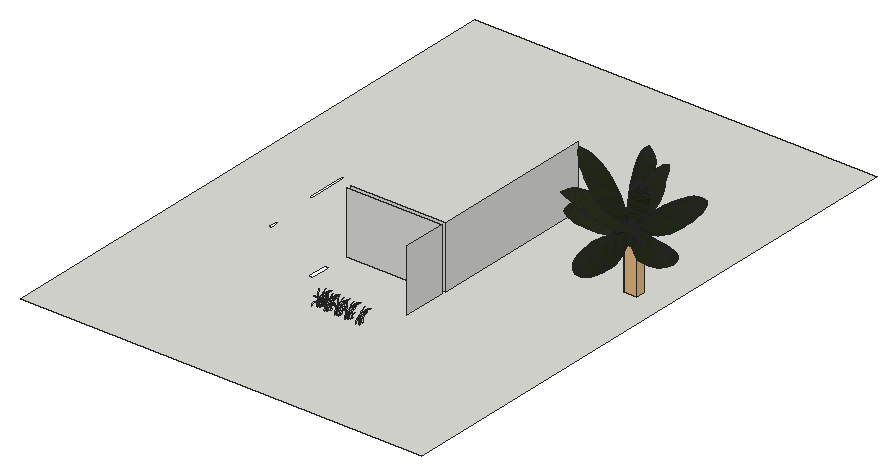
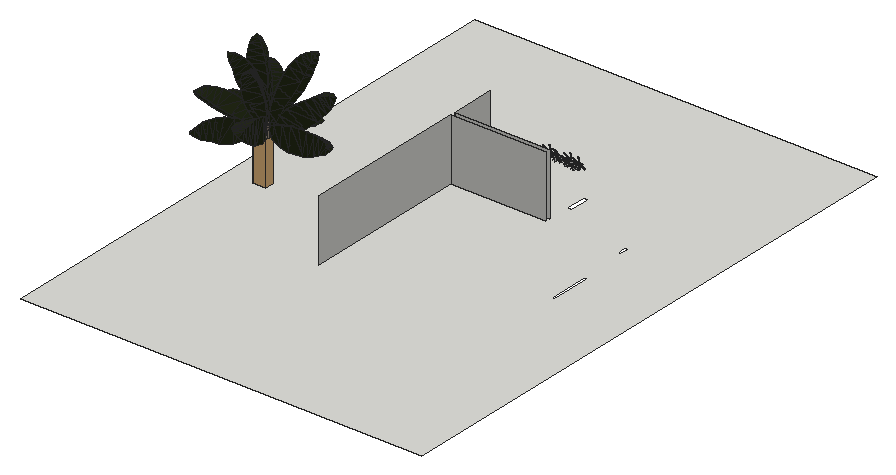
# SketchUp Ruby script. Lengths in inches.
U = 1.inch
M = Sketchup.active_model
def pt(a) = Geom::Point3d.new(a.map { |v| v * U })
def face(e, loops, mat)
  f = e.add_face(loops[0].map { |a| pt(a) })
  loops[1..].each { |l| e.add_face(l.map { |a| pt(a) }).erase! }
  f.material = f.back_material = mat if mat
  f
end
# faces: each face lists its corners as indices into pts; further lists are holes
def faces(e, pts, list, mat = nil) = list.each { |f| face(e, (f[0].is_a?(Array) ? f : [f]).map { |l| l.map { |i| pts[i] } }, mat) }
# xy, xz, yz: faces in a plane at the given z, y or x. An outline is a flat list of corners, or four numbers for a rectangle; further outlines are holes
def ring(l) = l.size == 4 ? [[l[0], l[1]], [l[2], l[1]], [l[2], l[3]], [l[0], l[3]]] : l.each_slice(2).to_a
def flat(e, list, mat, &to3) = list.each { |f| face(e, (f[0].is_a?(Array) ? f : [f]).map { |l| ring(l).map { |u, v| to3.(u, v) } }, mat) }
def xy(e, z, list, mat = nil) = flat(e, list, mat) { |x, y| [x, y, z] }
def xz(e, y, list, mat = nil) = flat(e, list, mat) { |x, z| [x, y, z] }
def yz(e, x, list, mat = nil) = flat(e, list, mat) { |y, z| [x, y, z] }
def lines(e, pts, list) = list.each { |a, b| e.add_line(pt(pts[a]), pt(pts[b])) }
# prism: a flat outline (further loops are holes) pulled along v
def prism(e, loops, v, mat = nil)
  f = face(e, loops, mat); d = Geom::Vector3d.new(v.map { |x| x * U })
  f.pushpull(f.normal.samedirection?(d) ? d.length : -d.length)
end
def box(e, o, s, mat = nil) = prism(e, [[o, [o[0] + s[0], o[1], o[2]], [o[0] + s[0], o[1] + s[1], o[2]], [o[0], o[1] + s[1], o[2]]]], [0, 0, s[2]], mat)
def at(x, y, z, deg = 0) = Geom::Transformation.translation(pt([x, y, z])) * Geom::Transformation.rotation(ORIGIN, Z_AXIS, deg.degrees)
def axes(o, x, y, z) = Geom::Transformation.new([*x, 0, *y, 0, *z, 0, *pt(o).to_a, 1])
def part(name) = M.definitions.add(name)
# library, detail: a bought-in or finely detailed component or shape, given as its bounding box
def library(name, o, s) = part(name).tap { |d| box(d.entities, o, s) }
def detail(e, o, s) = box(e.add_group.entities, o, s)
def put(e, d, t, mat = nil) = e.add_instance(d, t).tap { |i| i.material = mat if mat }
def group(e, t, mat = nil) = e.add_group.tap { |g| g.transformation = t; g.material = mat if mat }.entities
root = M.entities
M.materials.add("cocoanut_mat").color = [137, 122, 109]
M.materials.add("cocoanut_scrub").color = [165, 152, 134]
M.materials.add("coconut_test3_clean").color = [38, 45, 24]
c1 = part("coconut_half")
p = [[54.48,2.6,2.17],[90.24,0,0],[105.09,35.75,42.48],[115.87,5,0],[128.48,35.75,36.0625],[152.37,21,0],
  [152.37,35.75,27.13],[169.19,35.75,17.77],[57.93,35.75,46.59],[42.36,5.25,5.16],[79.93,35.75,46.59],[41.85,35.75,44.23],
  [28.04,8.5,7.49],[27.85,35.75,39.58],[16.59,14.5,9.63],[9.27,35.75,26.98],[6.26,23.5,11.78],[16.71,35.75,32.89],
  [0,35.75,14.25]]
faces(c1.entities,p,[[0,1,2],[1,3,4],[1,4,2],[3,5,6],[3,6,4],[5,7,6],[0,8,9],[0,10,8],
  [0,2,10],[9,11,12],[9,8,11],[12,13,14],[12,11,13],[14,15,16],[14,17,15],[14,13,17],
  [18,16,15]],"coconut_test3_clean")
c2 = part("Group\#44")
put(c2.entities,c1,at(0,0,0))
put(c2.entities,c1,axes([0,71.5,0],[1,0,0],[0,-1,0],[0,0,1]))
c3 = part("coconut3_top")
put(c3.entities,c2,axes([-176.42,-40.5625,245.57],[1,0,0],[0,0.96593,-0.25882],[0,0.25882,0.96593]))
g1 = group(c3.entities,at(-4.7,-151.6,178.32))
put(g1,c1,axes([0,0,0],[0.14944,0.9543,0.25882],[-0.87562,0.00613,0.48296],[0.4593,-0.2988,0.83652]))
put(g1,c1,axes([-62.61,0.4375,34.53],[0.14944,0.9543,0.25882],[0.87562,-0.00613,-0.48296],[0.4593,-0.2988,0.83652]))
put(c3.entities,c2,axes([171.02,-15.64,245.06],[-0.94665,0.32227,0],[-0.31128,-0.91439,-0.25882],[-0.08341,-0.24501,0.96593]))
put(c3.entities,c2,axes([41.29,183.8,264.73],[-0.39574,-0.90582,-0.15126],[0.91636,-0.40035,0],[-0.06056,-0.13861,0.98849]))
put(c3.entities,c2,axes([-77.19,156.92,280.49],[0.30009,-0.91813,-0.25882],[0.86338,0.14605,0.48296],[-0.40562,-0.36839,0.83652]))
put(c3.entities,c2,axes([-112.56,-104.35,340.4],[0.76036,0.41456,-0.5],[-0.63406,0.64068,-0.43301],[0.14083,0.64627,0.75]))
put(c3.entities,c2,axes([119.49,-113.07,311.83],[-0.54618,0.67208,-0.5],[-0.83762,-0.43208,0.3342],[0.00857,0.60135,0.79894]))
put(c3.entities,c2,axes([103.27,116.54,337.13],[-0.75167,-0.49748,-0.43301],[0.65951,-0.56129,-0.5],[0.0057,-0.66141,0.75]))
put(c3.entities,c2,axes([-111.91,-75.47,434.48],[0.55528,0.30275,-1.09544],[-0.10884,0.68367,0.13377],[0.95166,0.05419,0.49738]))
put(c3.entities,c2,axes([96.22,-37.8,421.8],[-0.43628,0.34579,-0.96422],[-0.35338,-0.74638,-0.10777],[-0.75439,0.29273,0.44631]))
put(c3.entities,c2,axes([-41.59,80.66,420.02],[0.06101,-0.43197,-0.99256],[0.722,0.18761,-0.03727],[0.23024,-0.81295,0.36796]))
put(c3.entities,c2,axes([62.57,69.42,421.8],[-0.49424,-0.25619,-0.96422],[0.53593,-0.62829,-0.10777],[-0.57624,-0.5681,0.44631]))
c4 = part("cocoanut_mat")
yz(c4.entities,2,[[0.45,5,4.17,5,4.55,7.22,0,7.22]],"cocoanut_mat")
p = [[1.5,0.95,2.55],[0,1.26,0],[1.5,4.17,2.55],[0,3.01,0.06],[2,0.45,5],[2,4.17,5],
  [1.5,4.82,10.82],[1.5,0,9.97],[2,4.55,7.22],[2,0,7.22],[1,0.99,11.1],[1,3.98,11.36]]
faces(c4.entities,p,[[0,1,2],[3,2,1],[4,0,2,5],[6,7,8],[9,8,7],[7,6,10],[11,10,6]],"cocoanut_mat")
c5 = part("Coconut Palm")
xy(c5.entities,112.14,[[122.28,106.09,125.08,107.25,126.24,110.05,125.08,112.85,122.28,114.01,119.48,112.85,118.32,110.05,119.48,107.25]])
detail(c5.entities,[118.32,101.24,0],[25.61,17.45,83.17])
put(c5.entities,c3,axes([125.26,110.5,-76.06],[0.71,0,0],[0,0.71,0],[0,0,0.71]))
g2 = group(c5.entities,at(117.6,103.69,82.125))
p = [[4.68,2.4,1.05],[4.68,2.4,30.02],[1.88,3.56,30.02],[1.88,3.56,1.05],[7.48,3.56,1.05],[7.48,3.56,30.02],
  [0.72,6.36,30.02],[0.72,6.36,1.05],[8.64,6.36,1.05],[8.64,6.36,30.02],[1.88,9.16,30.02],[1.88,9.16,1.05],
  [7.48,9.16,1.05],[7.48,9.16,30.02],[4.68,10.32,30.02],[4.68,10.32,1.05]]
faces(g2,p,[[0,1,2,3],[4,5,1,0],[2,6,7,3],[4,8,9,5],[6,10,11,7],[8,12,13,9],[11,10,14,15],[15,14,13,12]],"cocoanut_scrub")
put(g2,c4,axes([8.73,9,14.81],[0.95137,0.17914,0.2506],[-0.24236,0.93742,0.25],[-0.19013,-0.29858,0.93525]))
put(g2,c4,axes([1.89,13.92,14.26],[-0.95388,0.23795,0.18301],[-0.27087,-0.94506,-0.18301],[0.17341,-0.30035,1.29434]))
put(g2,c4,axes([3.98,0.08,4.09],[0.521,-0.82169,0.23104],[0.85353,0.50368,-0.13339],[-0.00676,0.2667,0.96376]))
put(g2,c4,axes([2.8,2.4,6.76],[-0.16755,-0.98247,0.08171],[0.984,-0.16156,0.07513],[-0.09879,0.15157,1.61993]))
put(g2,c4,axes([8.29,10.47,4.97],[0.02489,0.99575,0.08868],[-0.99708,0.03112,-0.06968],[-0.11254,-0.13523,1.55005]))
put(g2,c4,axes([10.54,2.88,6.76],[0.95137,0.17914,0.2506],[-0.115,0.96125,-0.25056],[-0.28577,0.20956,0.9351]))
xy(root,0,[[[75.43,0,853.18,1102.0625],[219.74,518.03,227.09,597.83],[372.21,325.52,381.21,367.52],[229.21,408.6,235.21,426.23]]])
xz(root,409.52,[[381.21,0,565.21,120]])
xz(root,418.52,[[381.21,0,565.21,120]])
yz(root,565.21,[[325.52,0,409.52,120],[418.52,0,739.58,120]])
g3 = group(root,at(460.01,260.65,0))
p = [[-0.98,0.17,0],[-0.43,0.08,0],[0,0,1.75],[-0.18,0.03,3.51],[-0.96,0.17,5.24],[-2.32,0.41,6.89],
  [-4.24,0.76,8.42],[-6.67,1.1875,9.8],[-9.54,1.7,10.98],[-12.78,2.28,11.95],[-16.32,2.91,12.67],[-20.06,3.57,13.13],
  [-23.91,4.26,13.32],[-27.78,4.95,13.23],[-23.98,4.27,13.25],[-20.22,3.6,13],[-16.59,2.96,12.5],[-13.16,2.34,11.75],
  [-10.02,1.79,10.78],[-7.25,1.29,9.6],[-4.89,0.87,8.25],[-3.02,0.54,6.75],[-1.66,0.3,5.13],[-0.86,0.15,3.44],
  [-0.63,0.11,1.72]]
faces(g3,p,[[0,1,2,3,4,5,6,7,8,9,10,11,12,13,14,15,16,17,18,19,20,21,22,23,24]])
g4 = group(root,at(460.01,260.65,0))
p = [[-0.98,0.17,0],[-0.43,0.08,0],[0,0,1.75],[-0.18,0.03,3.51],[-0.96,0.17,5.24],[-2.32,0.41,6.89],
  [-4.24,0.76,8.42],[-6.67,1.1875,9.8],[-9.54,1.7,10.98],[-12.78,2.28,11.95],[-16.32,2.91,12.67],[-20.06,3.57,13.13],
  [-23.91,4.26,13.32],[-27.78,4.95,13.23],[-23.98,4.27,13.25],[-20.22,3.6,13],[-16.59,2.96,12.5],[-13.16,2.34,11.75],
  [-10.02,1.79,10.78],[-7.25,1.29,9.6],[-4.89,0.87,8.25],[-3.02,0.54,6.75],[-1.66,0.3,5.13],[-0.86,0.15,3.44],
  [-0.63,0.11,1.72]]
faces(g4,p,[[0,1,2,3,4,5,6,7,8,9,10,11,12,13,14,15,16,17,18,19,20,21,22,23,24]])
g5 = group(root,at(499.26,259.53,0))
p = [[-0.4,0.86,0],[-0.18,0.38,2.26],[-0.05,0.1,4.55],[0,0,6.84],[-0.04,0.09,9.14],[-0.18,0.38,11.42],
  [-0.4,0.85,13.6875],[-0.71,1.51,15.92],[-1.1,2.36,18.12],[-1.58,3.38,20.26],[-2.14,4.58,22.35],[-2.79,5.95,24.37],
  [-3.51,7.48,26.3125],[-2.83,6.04,24.34],[-2.22,4.75,22.3],[-1.69,3.61,20.2],[-1.23,2.63,18.05],[-0.85,1.82,15.86],
  [-0.55,1.17,13.64],[-0.32,0.6875,11.38],[-0.18,0.38,9.11],[-0.11,0.24,6.83],[-0.13,0.28,4.54],[-0.23,0.48,2.27]]
faces(g5,p,[[0,1,2,3,4,5,6,7,8,9,10,11,12,13,14,15,16,17,18,19,20,21,22,23]])
g6 = group(root,at(459.13,259.55,0))
p = [[-0.4,0.86,0],[-0.18,0.38,2.26],[-0.05,0.1,4.55],[0,0,6.84],[-0.04,0.09,9.14],[-0.18,0.38,11.42],
  [-0.4,0.85,13.6875],[-0.71,1.51,15.92],[-1.1,2.36,18.12],[-1.58,3.38,20.26],[-2.14,4.58,22.35],[-2.79,5.95,24.37],
  [-3.51,7.48,26.3125],[-2.83,6.04,24.34],[-2.22,4.75,22.3],[-1.69,3.61,20.2],[-1.23,2.63,18.05],[-0.85,1.82,15.86],
  [-0.55,1.17,13.64],[-0.32,0.6875,11.38],[-0.18,0.38,9.11],[-0.11,0.24,6.83],[-0.13,0.28,4.54],[-0.23,0.48,2.27]]
faces(g6,p,[[0,1,2,3,4,5,6,7,8,9,10,11,12,13,14,15,16,17,18,19,20,21,22,23]])
g7 = group(root,at(482.85,258.46,0))
p = [[-0.62,0.44,0],[-0.27,0.2,0],[0,0,1.68],[-0.11,0.08,3.37],[-0.6,0.43,5.03],[-1.46,1.05,6.61],
  [-2.67,1.92,8.08],[-4.2,3.02,9.4],[-6.01,4.32,10.54],[-8.05,5.79,11.47],[-10.28,7.39,12.16],[-12.64,9.08,12.61],
  [-15.07,10.83,12.79],[-17.5,12.58,12.7],[-15.11,10.86,12.72],[-12.74,9.16,12.48],[-10.45,7.51,12],[-8.29,5.96,11.29],
  [-6.32,4.54,10.35],[-4.57,3.28,9.22],[-3.08,2.21,7.92],[-1.9,1.37,6.48],[-1.05,0.75,4.93],[-0.54,0.39,3.31],
  [-0.4,0.29,1.65]]
faces(g7,p,[[0,1,2,3,4,5,6,7,8,9,10,11,12,13,14,15,16,17,18,19,20,21,22,23,24]])
g8 = group(root,at(479.6,261.04,0))
p = [[7.51,7.51,22.54],[6.3125,6.3125,20.88],[5.21,5.21,19.16],[4.21,4.21,17.39],[3.32,3.32,15.57],[2.52,2.52,13.71],
  [1.84,1.84,11.82],[1.27,1.27,9.89],[0.81,0.81,7.94],[0.46,0.46,5.97],[0.22,0.22,3.99],[0.1,0.1,2],
  [0.1,0.1,0],[0,0,2.01],[0.04,0.04,4.01],[0.21,0.21,6.01],[0.51,0.51,8],[0.95,0.95,9.97],
  [1.51,1.51,11.91],[2.21,2.21,13.81],[3.03,3.03,15.67],[3.98,3.98,17.48],[5.04,5.04,19.23],[6.22,6.22,20.92]]
faces(g8,p,[[0,1,2,3,4,5,6,7,8,9,10,11,12,13,14,15,16,17,18,19,20,21,22,23]])
g9 = group(root,at(483.02,259.85,0))
p = [[-0.93,0.35,0],[-0.41,0.16,0],[0,0,1.75],[-0.17,0.0625,3.51],[-0.91,0.34,5.24],[-2.21,0.83,6.89],
  [-4.03,1.52,8.42],[-6.34,2.39,9.8],[-9.0625,3.42,10.98],[-12.14,4.59,11.95],[-15.5,5.86,12.67],[-19.06,7.2,13.13],
  [-22.72,8.58,13.32],[-26.4,9.97,13.23],[-22.79,8.61,13.25],[-19.22,7.26,13],[-15.76,5.96,12.5],[-12.51,4.73,11.75],
  [-9.53,3.6,10.78],[-6.89,2.6,9.6],[-4.65,1.76,8.25],[-2.87,1.08,6.75],[-1.58,0.6,5.13],[-0.82,0.31,3.44],
  [-0.6,0.23,1.72]]
faces(g9,p,[[0,1,2,3,4,5,6,7,8,9,10,11,12,13,14,15,16,17,18,19,20,21,22,23,24]])
g10 = group(root,at(484.06,262.77,0))
p = [[5.08,5.08,9.0625],[4.15,4.15,8.49],[3.31,3.31,7.85],[2.57,2.57,7.18],[1.93,1.93,6.45],[1.41,1.41,5.7],
  [0.99,0.99,4.91],[0.7,0.7,4.1],[0.53,0.53,3.28],[0.48,0.48,2.45],[0.55,0.55,1.625],[0.75,0.75,0.8],
  [1.0625,1.0625,0],[0.65,0.65,0],[0.3,0.3,0.81],[0.08,0.08,1.65],[0,0,2.49],[0.06,0.06,3.34],
  [0.25,0.25,4.17],[0.58,0.58,4.99],[1.04,1.04,5.79],[1.62,1.62,6.54],[2.33,2.33,7.26],[3.14,3.14,7.92],
  [4.0625,4.0625,8.52]]
faces(g10,p,[[0,1,2,3,4,5,6,7,8,9,10,11,12,13,14,15,16,17,18,19,20,21,22,23,24]])
g11 = group(root,at(433.07,258.71,0))
p = [[17.17,11.7,12.375],[19.76,13.47,12.7],[17.25,11.76,12.31],[14.83,10.11,11.76],[12.52,8.53,11.07],[10.35,7.05,10.23],
  [8.34,5.68,9.27],[6.52,4.44,8.2],[4.9,3.34,7.01],[3.51,2.39,5.74],[2.35,1.6,4.38],[1.45,0.99,2.96],
  [0.82,0.56,1.5],[0.45,0.3,0],[0,0,0],[0.3,0.21,1.53],[0.9,0.61,3.03],[1.78,1.22,4.49],
  [2.95,2.01,5.875],[4.37,2.98,7.18],[6.03,4.11,8.375],[7.92,5.4,9.46],[10,6.82,10.41],[12.26,8.36,11.22],
  [14.66,9.99,11.88]]
faces(g11,p,[[0,1,2,3,4,5,6,7,8,9,10,11,12,13,14,15,16,17,18,19,20,21,22,23,24]])
g12 = group(root,at(502.33,259.2,0))
p = [[-0.62,0.44,0],[-0.27,0.2,0],[0,0,1.68],[-0.11,0.08,3.37],[-0.6,0.43,5.03],[-1.46,1.05,6.61],
  [-2.67,1.92,8.08],[-4.2,3.02,9.4],[-6.01,4.32,10.54],[-8.05,5.79,11.47],[-10.28,7.39,12.16],[-12.64,9.08,12.61],
  [-15.07,10.83,12.79],[-17.5,12.58,12.7],[-15.11,10.86,12.72],[-12.74,9.16,12.48],[-10.45,7.51,12],[-8.29,5.96,11.29],
  [-6.32,4.54,10.35],[-4.57,3.28,9.22],[-3.08,2.21,7.92],[-1.9,1.37,6.48],[-1.05,0.75,4.93],[-0.54,0.39,3.31],
  [-0.4,0.29,1.65]]
faces(g12,p,[[0,1,2,3,4,5,6,7,8,9,10,11,12,13,14,15,16,17,18,19,20,21,22,23,24]])
g13 = group(root,at(462.19,259.22,0))
p = [[-0.62,0.44,0],[-0.27,0.2,0],[0,0,1.68],[-0.11,0.08,3.37],[-0.6,0.43,5.03],[-1.46,1.05,6.61],
  [-2.67,1.92,8.08],[-4.2,3.02,9.4],[-6.01,4.32,10.54],[-8.05,5.79,11.47],[-10.28,7.39,12.16],[-12.64,9.08,12.61],
  [-15.07,10.83,12.79],[-17.5,12.58,12.7],[-15.11,10.86,12.72],[-12.74,9.16,12.48],[-10.45,7.51,12],[-8.29,5.96,11.29],
  [-6.32,4.54,10.35],[-4.57,3.28,9.22],[-3.08,2.21,7.92],[-1.9,1.37,6.48],[-1.05,0.75,4.93],[-0.54,0.39,3.31],
  [-0.4,0.29,1.65]]
faces(g13,p,[[0,1,2,3,4,5,6,7,8,9,10,11,12,13,14,15,16,17,18,19,20,21,22,23,24]])
g14 = group(root,at(499.07,261.78,0))
p = [[7.51,7.51,22.54],[6.3125,6.3125,20.88],[5.21,5.21,19.16],[4.21,4.21,17.39],[3.32,3.32,15.57],[2.52,2.52,13.71],
  [1.84,1.84,11.82],[1.27,1.27,9.89],[0.81,0.81,7.94],[0.46,0.46,5.97],[0.22,0.22,3.99],[0.1,0.1,2],
  [0.1,0.1,0],[0,0,2.01],[0.04,0.04,4.01],[0.21,0.21,6.01],[0.51,0.51,8],[0.95,0.95,9.97],
  [1.51,1.51,11.91],[2.21,2.21,13.81],[3.03,3.03,15.67],[3.98,3.98,17.48],[5.04,5.04,19.23],[6.22,6.22,20.92]]
faces(g14,p,[[0,1,2,3,4,5,6,7,8,9,10,11,12,13,14,15,16,17,18,19,20,21,22,23]])
g15 = group(root,at(458.9375,261.8,0))
p = [[7.51,7.51,22.54],[6.3125,6.3125,20.88],[5.21,5.21,19.16],[4.21,4.21,17.39],[3.32,3.32,15.57],[2.52,2.52,13.71],
  [1.84,1.84,11.82],[1.27,1.27,9.89],[0.81,0.81,7.94],[0.46,0.46,5.97],[0.22,0.22,3.99],[0.1,0.1,2],
  [0.1,0.1,0],[0,0,2.01],[0.04,0.04,4.01],[0.21,0.21,6.01],[0.51,0.51,8],[0.95,0.95,9.97],
  [1.51,1.51,11.91],[2.21,2.21,13.81],[3.03,3.03,15.67],[3.98,3.98,17.48],[5.04,5.04,19.23],[6.22,6.22,20.92]]
faces(g15,p,[[0,1,2,3,4,5,6,7,8,9,10,11,12,13,14,15,16,17,18,19,20,21,22,23]])
g16 = group(root,at(443.27,261.24,0))
p = [[-3.85,8.68,9.0625],[-3.11,7.03,8.49],[-2.45,5.54,7.85],[-1.87,4.22,7.18],[-1.37,3.08,6.45],[-0.95,2.15,5.7],
  [-0.625,1.41,4.91],[-0.39,0.89,4.1],[-0.26,0.58,3.28],[-0.22,0.49,2.45],[-0.28,0.625,1.625],[-0.43,0.97,0.8],
  [-0.68,1.54,0],[-0.52,1.16,0],[-0.23,0.52,0.8],[-0.05,0.11,1.61],[0.02,-0.06,2.45],[-0.01,0.02,3.28],
  [-0.15,0.33,4.11],[-0.39,0.89,4.93],[-0.74,1.67,5.72],[-1.1875,2.68,6.49],[-1.73,3.9,7.21],[-2.35,5.3125,7.88],
  [-3.0625,6.91,8.5]]
faces(g16,p,[[0,1,2,3,4,5,6,7,8,9,10,11,12,13,14,15,16,17,18,19,20,21,22,23,24]])
g17 = group(root,at(502.49,260.59,0))
p = [[-0.93,0.35,0],[-0.41,0.16,0],[0,0,1.75],[-0.17,0.0625,3.51],[-0.91,0.34,5.24],[-2.21,0.83,6.89],
  [-4.03,1.52,8.42],[-6.34,2.39,9.8],[-9.0625,3.42,10.98],[-12.14,4.59,11.95],[-15.5,5.86,12.67],[-19.06,7.2,13.13],
  [-22.72,8.58,13.32],[-26.4,9.97,13.23],[-22.79,8.61,13.25],[-19.22,7.26,13],[-15.76,5.96,12.5],[-12.51,4.73,11.75],
  [-9.53,3.6,10.78],[-6.89,2.6,9.6],[-4.65,1.76,8.25],[-2.87,1.08,6.75],[-1.58,0.6,5.13],[-0.82,0.31,3.44],
  [-0.6,0.23,1.72]]
faces(g17,p,[[0,1,2,3,4,5,6,7,8,9,10,11,12,13,14,15,16,17,18,19,20,21,22,23,24]])
g18 = group(root,at(462.36,260.61,0))
p = [[-0.93,0.35,0],[-0.41,0.16,0],[0,0,1.75],[-0.17,0.0625,3.51],[-0.91,0.34,5.24],[-2.21,0.83,6.89],
  [-4.03,1.52,8.42],[-6.34,2.39,9.8],[-9.0625,3.42,10.98],[-12.14,4.59,11.95],[-15.5,5.86,12.67],[-19.06,7.2,13.13],
  [-22.72,8.58,13.32],[-26.4,9.97,13.23],[-22.79,8.61,13.25],[-19.22,7.26,13],[-15.76,5.96,12.5],[-12.51,4.73,11.75],
  [-9.53,3.6,10.78],[-6.89,2.6,9.6],[-4.65,1.76,8.25],[-2.87,1.08,6.75],[-1.58,0.6,5.13],[-0.82,0.31,3.44],
  [-0.6,0.23,1.72]]
faces(g18,p,[[0,1,2,3,4,5,6,7,8,9,10,11,12,13,14,15,16,17,18,19,20,21,22,23,24]])
g19 = group(root,at(441.82,262.2,0))
p = [[-0.4,0.86,0],[-0.18,0.38,2.26],[-0.05,0.1,4.55],[0,0,6.84],[-0.04,0.09,9.14],[-0.18,0.38,11.42],
  [-0.4,0.85,13.6875],[-0.71,1.51,15.92],[-1.1,2.36,18.12],[-1.58,3.38,20.26],[-2.14,4.58,22.35],[-2.79,5.95,24.37],
  [-3.51,7.48,26.3125],[-2.83,6.04,24.34],[-2.22,4.75,22.3],[-1.69,3.61,20.2],[-1.23,2.63,18.05],[-0.85,1.82,15.86],
  [-0.55,1.17,13.64],[-0.32,0.6875,11.38],[-0.18,0.38,9.11],[-0.11,0.24,6.83],[-0.13,0.28,4.54],[-0.23,0.48,2.27]]
faces(g19,p,[[0,1,2,3,4,5,6,7,8,9,10,11,12,13,14,15,16,17,18,19,20,21,22,23]])
g20 = group(root,at(503.53,263.51,0))
p = [[5.08,5.08,9.0625],[4.15,4.15,8.49],[3.31,3.31,7.85],[2.57,2.57,7.18],[1.93,1.93,6.45],[1.41,1.41,5.7],
  [0.99,0.99,4.91],[0.7,0.7,4.1],[0.53,0.53,3.28],[0.48,0.48,2.45],[0.55,0.55,1.625],[0.75,0.75,0.8],
  [1.0625,1.0625,0],[0.65,0.65,0],[0.3,0.3,0.81],[0.08,0.08,1.65],[0,0,2.49],[0.06,0.06,3.34],
  [0.25,0.25,4.17],[0.58,0.58,4.99],[1.04,1.04,5.79],[1.62,1.62,6.54],[2.33,2.33,7.26],[3.14,3.14,7.92],
  [4.0625,4.0625,8.52]]
faces(g20,p,[[0,1,2,3,4,5,6,7,8,9,10,11,12,13,14,15,16,17,18,19,20,21,22,23,24]])
g21 = group(root,at(527.45,263.52,0))
p = [[5.08,5.08,18.42],[4.15,4.15,17.25],[3.31,3.31,15.97],[2.57,2.57,14.59],[1.93,1.93,13.12],[1.41,1.41,11.58],
  [0.99,0.99,9.98],[0.7,0.7,8.34],[0.53,0.53,6.67],[0.48,0.48,4.99],[0.55,0.55,3.3],[0.75,0.75,1.63],
  [1.0625,1.0625,0],[0.65,0.65,0],[0.3,0.3,1.66],[0.08,0.08,3.35],[0,0,5.07],[0.06,0.06,6.79],
  [0.25,0.25,8.49],[0.58,0.58,10.15],[1.04,1.04,11.76],[1.62,1.62,13.3],[2.33,2.33,14.75],[3.14,3.14,16.1],
  [4.0625,4.0625,17.33]]
faces(g21,p,[[0,1,2,3,4,5,6,7,8,9,10,11,12,13,14,15,16,17,18,19,20,21,22,23,24]])
g22 = group(root,at(463.4,263.52,0))
p = [[5.08,5.08,9.0625],[4.15,4.15,8.49],[3.31,3.31,7.85],[2.57,2.57,7.18],[1.93,1.93,6.45],[1.41,1.41,5.7],
  [0.99,0.99,4.91],[0.7,0.7,4.1],[0.53,0.53,3.28],[0.48,0.48,2.45],[0.55,0.55,1.625],[0.75,0.75,0.8],
  [1.0625,1.0625,0],[0.65,0.65,0],[0.3,0.3,0.81],[0.08,0.08,1.65],[0,0,2.49],[0.06,0.06,3.34],
  [0.25,0.25,4.17],[0.58,0.58,4.99],[1.04,1.04,5.79],[1.62,1.62,6.54],[2.33,2.33,7.26],[3.14,3.14,7.92],
  [4.0625,4.0625,8.52]]
faces(g22,p,[[0,1,2,3,4,5,6,7,8,9,10,11,12,13,14,15,16,17,18,19,20,21,22,23,24]])
g23 = group(root,at(441.625,264.45,0))
p = [[7.51,7.51,22.54],[6.3125,6.3125,20.88],[5.21,5.21,19.16],[4.21,4.21,17.39],[3.32,3.32,15.57],[2.52,2.52,13.71],
  [1.84,1.84,11.82],[1.27,1.27,9.89],[0.81,0.81,7.94],[0.46,0.46,5.97],[0.22,0.22,3.99],[0.1,0.1,2],
  [0.1,0.1,0],[0,0,2.01],[0.04,0.04,4.01],[0.21,0.21,6.01],[0.51,0.51,8],[0.95,0.95,9.97],
  [1.51,1.51,11.91],[2.21,2.21,13.81],[3.03,3.03,15.67],[3.98,3.98,17.48],[5.04,5.04,19.23],[6.22,6.22,20.92]]
faces(g23,p,[[0,1,2,3,4,5,6,7,8,9,10,11,12,13,14,15,16,17,18,19,20,21,22,23]])
g24 = group(root,at(484.4,265.84,0))
p = [[5.08,5.08,18.42],[4.15,4.15,17.25],[3.31,3.31,15.97],[2.57,2.57,14.59],[1.93,1.93,13.12],[1.41,1.41,11.58],
  [0.99,0.99,9.98],[0.7,0.7,8.34],[0.53,0.53,6.67],[0.48,0.48,4.99],[0.55,0.55,3.3],[0.75,0.75,1.63],
  [1.0625,1.0625,0],[0.65,0.65,0],[0.3,0.3,1.66],[0.08,0.08,3.35],[0,0,5.07],[0.06,0.06,6.79],
  [0.25,0.25,8.49],[0.58,0.58,10.15],[1.04,1.04,11.76],[1.62,1.62,13.3],[2.33,2.33,14.75],[3.14,3.14,16.1],
  [4.0625,4.0625,17.33]]
faces(g24,p,[[0,1,2,3,4,5,6,7,8,9,10,11,12,13,14,15,16,17,18,19,20,21,22,23,24]])
g25 = group(root,at(446.08,266.18,0))
p = [[5.08,5.08,9.0625],[4.15,4.15,8.49],[3.31,3.31,7.85],[2.57,2.57,7.18],[1.93,1.93,6.45],[1.41,1.41,5.7],
  [0.99,0.99,4.91],[0.7,0.7,4.1],[0.53,0.53,3.28],[0.48,0.48,2.45],[0.55,0.55,1.625],[0.75,0.75,0.8],
  [1.0625,1.0625,0],[0.65,0.65,0],[0.3,0.3,0.81],[0.08,0.08,1.65],[0,0,2.49],[0.06,0.06,3.34],
  [0.25,0.25,4.17],[0.58,0.58,4.99],[1.04,1.04,5.79],[1.62,1.62,6.54],[2.33,2.33,7.26],[3.14,3.14,7.92],
  [4.0625,4.0625,8.52]]
faces(g25,p,[[0,1,2,3,4,5,6,7,8,9,10,11,12,13,14,15,16,17,18,19,20,21,22,23,24]])
g26 = group(root,at(503.87,266.58,0))
p = [[5.08,5.08,18.42],[4.15,4.15,17.25],[3.31,3.31,15.97],[2.57,2.57,14.59],[1.93,1.93,13.12],[1.41,1.41,11.58],
  [0.99,0.99,9.98],[0.7,0.7,8.34],[0.53,0.53,6.67],[0.48,0.48,4.99],[0.55,0.55,3.3],[0.75,0.75,1.63],
  [1.0625,1.0625,0],[0.65,0.65,0],[0.3,0.3,1.66],[0.08,0.08,3.35],[0,0,5.07],[0.06,0.06,6.79],
  [0.25,0.25,8.49],[0.58,0.58,10.15],[1.04,1.04,11.76],[1.62,1.62,13.3],[2.33,2.33,14.75],[3.14,3.14,16.1],
  [4.0625,4.0625,17.33]]
faces(g26,p,[[0,1,2,3,4,5,6,7,8,9,10,11,12,13,14,15,16,17,18,19,20,21,22,23,24]])
g27 = group(root,at(463.74,266.6,0))
p = [[5.08,5.08,18.42],[4.15,4.15,17.25],[3.31,3.31,15.97],[2.57,2.57,14.59],[1.93,1.93,13.12],[1.41,1.41,11.58],
  [0.99,0.99,9.98],[0.7,0.7,8.34],[0.53,0.53,6.67],[0.48,0.48,4.99],[0.55,0.55,3.3],[0.75,0.75,1.63],
  [1.0625,1.0625,0],[0.65,0.65,0],[0.3,0.3,1.66],[0.08,0.08,3.35],[0,0,5.07],[0.06,0.06,6.79],
  [0.25,0.25,8.49],[0.58,0.58,10.15],[1.04,1.04,11.76],[1.62,1.62,13.3],[2.33,2.33,14.75],[3.14,3.14,16.1],
  [4.0625,4.0625,17.33]]
faces(g27,p,[[0,1,2,3,4,5,6,7,8,9,10,11,12,13,14,15,16,17,18,19,20,21,22,23,24]])
g28 = group(root,at(521.72,255.23,0))
p = [[0.08,0.99,0],[0.03,0.44,0],[0,0,2.01],[0.01,0.18,4.04],[0.08,0.97,6.02],[0.19,2.35,7.92],
  [0.34,4.3,9.68],[0.53,6.75,11.26],[0.76,9.66,12.62],[1.02,12.94,13.73],[1.3,16.52,14.5625],[1.6,20.31,15.09],
  [1.91,24.21,15.31],[2.21,28.13,15.2],[1.91,24.29,15.22],[1.61,20.48,14.94],[1.32,16.8,14.37],[1.05,13.33,13.51],
  [0.8,10.15,12.39],[0.58,7.34,11.04],[0.39,4.95,9.48],[0.24,3.05,7.75],[0.13,1.68,5.9],[0.07,0.87,3.96],
  [0.05,0.64,1.98]]
faces(g28,p,[[0,1,2,3,4,5,6,7,8,9,10,11,12,13,14,15,16,17,18,19,20,21,22,23,24]])
g29 = group(root,at(527.18,256.94,0))
p = [[0.07,0.92,0],[0.03,0.41,0],[0,0,2.37],[0.01,0.17,4.75],[0.07,0.9,7.08],[0.17,2.19,9.32],
  [0.32,4,11.39],[0.5,6.29,13.25],[0.71,9,14.85],[0.95,12.06,16.15],[1.21,15.39,17.13],[1.49,18.92,17.75],
  [1.78,22.55,18.01],[2.0625,26.21,17.89],[1.78,22.625,17.91],[1.5,19.08,17.58],[1.23,15.65,16.9],[0.98,12.42,15.89],
  [0.74,9.46,14.58],[0.54,6.84,12.99],[0.36,4.61,11.15],[0.22,2.84,9.125],[0.125,1.57,6.94],[0.0625,0.8125,4.66],
  [0.05,0.59,2.33]]
faces(g29,p,[[0,1,2,3,4,5,6,7,8,9,10,11,12,13,14,15,16,17,18,19,20,21,22,23,24]])
g30 = group(root,at(481.38,259.74,0))
p = [[-0.5,0.78,0],[-0.22,0.34,0],[0,0,2.37],[-0.09,0.14,4.75],[-0.49,0.76,7.08],[-1.2,1.84,9.32],
  [-2.1875,3.37,11.39],[-3.4375,5.29,13.25],[-4.92,7.57,14.85],[-6.59,10.14,16.15],[-8.41,12.95,17.13],[-10.34,15.92,17.75],
  [-12.32,18.97,18.01],[-14.32,22.05,17.89],[-12.36,19.03,17.91],[-10.42,16.05,17.58],[-8.55,13.16,16.9],[-6.78,10.45,15.89],
  [-5.17,7.96,14.58],[-3.73,5.75,12.99],[-2.52,3.88,11.15],[-1.55,2.39,9.125],[-0.86,1.32,6.94],[-0.44,0.68,4.66],
  [-0.33,0.5,2.33]]
faces(g30,p,[[0,1,2,3,4,5,6,7,8,9,10,11,12,13,14,15,16,17,18,19,20,21,22,23,24]])
g31 = group(root,at(524.14,258.26,0))
p = [[-0.27,0.88,0],[-0.12,0.39,0],[0,0,2.0625],[-0.05,0.16,4.13],[-0.26,0.87,6.16],[-0.64,2.1,8.1],
  [-1.17,3.84,9.91],[-1.84,6.03,11.52],[-2.64,8.63,12.92],[-3.54,11.5625,14.05],[-4.51,14.76,14.9],[-5.55,18.15,15.45],
  [-6.61,21.64,15.67],[-7.69,25.14,15.5625],[-6.63,21.7,15.58],[-5.59,18.3,15.29],[-4.59,15.01,14.71],[-3.64,11.91,13.83],
  [-2.77,9.07,12.68],[-2,6.56,11.3],[-1.35,4.43,9.7],[-0.83,2.73,7.9375],[-0.46,1.5,6.04],[-0.24,0.78,4.05],
  [-0.17,0.57,2.02]]
faces(g31,p,[[0,1,2,3,4,5,6,7,8,9,10,11,12,13,14,15,16,17,18,19,20,21,22,23,24]])
g32 = group(root,at(460.72,260.5,0))
p = [[-0.5,0.78,0],[-0.22,0.34,0],[0,0,2.37],[-0.09,0.14,4.75],[-0.49,0.76,7.08],[-1.2,1.84,9.32],
  [-2.1875,3.37,11.39],[-3.4375,5.29,13.25],[-4.92,7.57,14.85],[-6.59,10.14,16.15],[-8.41,12.95,17.13],[-10.34,15.92,17.75],
  [-12.32,18.97,18.01],[-14.32,22.05,17.89],[-12.36,19.03,17.91],[-10.42,16.05,17.58],[-8.55,13.16,16.9],[-6.78,10.45,15.89],
  [-5.17,7.96,14.58],[-3.73,5.75,12.99],[-2.52,3.88,11.15],[-1.55,2.39,9.125],[-0.86,1.32,6.94],[-0.44,0.68,4.66],
  [-0.33,0.5,2.33]]
faces(g32,p,[[0,1,2,3,4,5,6,7,8,9,10,11,12,13,14,15,16,17,18,19,20,21,22,23,24]])
g33 = group(root,at(478.67,257.56,0))
p = [[0.08,0.99,0],[0.03,0.44,0],[0,0,2.01],[0.01,0.18,4.04],[0.08,0.97,6.02],[0.19,2.35,7.92],
  [0.34,4.3,9.68],[0.53,6.75,11.26],[0.76,9.66,12.62],[1.02,12.94,13.73],[1.3,16.52,14.5625],[1.6,20.31,15.09],
  [1.91,24.21,15.31],[2.21,28.13,15.2],[1.91,24.29,15.22],[1.61,20.48,14.94],[1.32,16.8,14.37],[1.05,13.33,13.51],
  [0.8,10.15,12.39],[0.58,7.34,11.04],[0.39,4.95,9.48],[0.24,3.05,7.75],[0.13,1.68,5.9],[0.07,0.87,3.96],
  [0.05,0.64,1.98]]
faces(g33,p,[[0,1,2,3,4,5,6,7,8,9,10,11,12,13,14,15,16,17,18,19,20,21,22,23,24]])
g34 = group(root,at(446.43,269.25,0))
p = [[5.08,5.08,18.42],[4.15,4.15,17.25],[3.31,3.31,15.97],[2.57,2.57,14.59],[1.93,1.93,13.12],[1.41,1.41,11.58],
  [0.99,0.99,9.98],[0.7,0.7,8.34],[0.53,0.53,6.67],[0.48,0.48,4.99],[0.55,0.55,3.3],[0.75,0.75,1.63],
  [1.0625,1.0625,0],[0.65,0.65,0],[0.3,0.3,1.66],[0.08,0.08,3.35],[0,0,5.07],[0.06,0.06,6.79],
  [0.25,0.25,8.49],[0.58,0.58,10.15],[1.04,1.04,11.76],[1.62,1.62,13.3],[2.33,2.33,14.75],[3.14,3.14,16.1],
  [4.0625,4.0625,17.33]]
faces(g34,p,[[0,1,2,3,4,5,6,7,8,9,10,11,12,13,14,15,16,17,18,19,20,21,22,23,24]])
g35 = group(root,at(498.14,258.29,0))
p = [[0.08,0.99,0],[0.03,0.44,0],[0,0,2.01],[0.01,0.18,4.04],[0.08,0.97,6.02],[0.19,2.35,7.92],
  [0.34,4.3,9.68],[0.53,6.75,11.26],[0.76,9.66,12.62],[1.02,12.94,13.73],[1.3,16.52,14.5625],[1.6,20.31,15.09],
  [1.91,24.21,15.31],[2.21,28.13,15.2],[1.91,24.29,15.22],[1.61,20.48,14.94],[1.32,16.8,14.37],[1.05,13.33,13.51],
  [0.8,10.15,12.39],[0.58,7.34,11.04],[0.39,4.95,9.48],[0.24,3.05,7.75],[0.13,1.68,5.9],[0.07,0.87,3.96],
  [0.05,0.64,1.98]]
faces(g35,p,[[0,1,2,3,4,5,6,7,8,9,10,11,12,13,14,15,16,17,18,19,20,21,22,23,24]])
g36 = group(root,at(484.13,259.27,0))
p = [[0.07,0.92,0],[0.03,0.41,0],[0,0,2.37],[0.01,0.17,4.75],[0.07,0.9,7.08],[0.17,2.19,9.32],
  [0.32,4,11.39],[0.5,6.29,13.25],[0.71,9,14.85],[0.95,12.06,16.15],[1.21,15.39,17.13],[1.49,18.92,17.75],
  [1.78,22.55,18.01],[2.0625,26.21,17.89],[1.78,22.625,17.91],[1.5,19.08,17.58],[1.23,15.65,16.9],[0.98,12.42,15.89],
  [0.74,9.46,14.58],[0.54,6.84,12.99],[0.36,4.61,11.15],[0.22,2.84,9.125],[0.125,1.57,6.94],[0.0625,0.8125,4.66],
  [0.05,0.59,2.33]]
faces(g36,p,[[0,1,2,3,4,5,6,7,8,9,10,11,12,13,14,15,16,17,18,19,20,21,22,23,24]])
g37 = group(root,at(458.01,258.3125,0))
p = [[0.08,0.99,0],[0.03,0.44,0],[0,0,2.01],[0.01,0.18,4.04],[0.08,0.97,6.02],[0.19,2.35,7.92],
  [0.34,4.3,9.68],[0.53,6.75,11.26],[0.76,9.66,12.62],[1.02,12.94,13.73],[1.3,16.52,14.5625],[1.6,20.31,15.09],
  [1.91,24.21,15.31],[2.21,28.13,15.2],[1.91,24.29,15.22],[1.61,20.48,14.94],[1.32,16.8,14.37],[1.05,13.33,13.51],
  [0.8,10.15,12.39],[0.58,7.34,11.04],[0.39,4.95,9.48],[0.24,3.05,7.75],[0.13,1.68,5.9],[0.07,0.87,3.96],
  [0.05,0.64,1.98]]
faces(g37,p,[[0,1,2,3,4,5,6,7,8,9,10,11,12,13,14,15,16,17,18,19,20,21,22,23,24]])
g38 = group(root,at(503.6,260,0))
p = [[0.07,0.92,0],[0.03,0.41,0],[0,0,2.37],[0.01,0.17,4.75],[0.07,0.9,7.08],[0.17,2.19,9.32],
  [0.32,4,11.39],[0.5,6.29,13.25],[0.71,9,14.85],[0.95,12.06,16.15],[1.21,15.39,17.13],[1.49,18.92,17.75],
  [1.78,22.55,18.01],[2.0625,26.21,17.89],[1.78,22.625,17.91],[1.5,19.08,17.58],[1.23,15.65,16.9],[0.98,12.42,15.89],
  [0.74,9.46,14.58],[0.54,6.84,12.99],[0.36,4.61,11.15],[0.22,2.84,9.125],[0.125,1.57,6.94],[0.0625,0.8125,4.66],
  [0.05,0.59,2.33]]
faces(g38,p,[[0,1,2,3,4,5,6,7,8,9,10,11,12,13,14,15,16,17,18,19,20,21,22,23,24]])
g39 = group(root,at(463.47,260.02,0))
p = [[0.07,0.92,0],[0.03,0.41,0],[0,0,2.37],[0.01,0.17,4.75],[0.07,0.9,7.08],[0.17,2.19,9.32],
  [0.32,4,11.39],[0.5,6.29,13.25],[0.71,9,14.85],[0.95,12.06,16.15],[1.21,15.39,17.13],[1.49,18.92,17.75],
  [1.78,22.55,18.01],[2.0625,26.21,17.89],[1.78,22.625,17.91],[1.5,19.08,17.58],[1.23,15.65,16.9],[0.98,12.42,15.89],
  [0.74,9.46,14.58],[0.54,6.84,12.99],[0.36,4.61,11.15],[0.22,2.84,9.125],[0.125,1.57,6.94],[0.0625,0.8125,4.66],
  [0.05,0.59,2.33]]
faces(g39,p,[[0,1,2,3,4,5,6,7,8,9,10,11,12,13,14,15,16,17,18,19,20,21,22,23,24]])
g40 = group(root,at(481.09,260.59,0))
p = [[-0.27,0.88,0],[-0.12,0.39,0],[0,0,2.0625],[-0.05,0.16,4.13],[-0.26,0.87,6.16],[-0.64,2.1,8.1],
  [-1.17,3.84,9.91],[-1.84,6.03,11.52],[-2.64,8.63,12.92],[-3.54,11.5625,14.05],[-4.51,14.76,14.9],[-5.55,18.15,15.45],
  [-6.61,21.64,15.67],[-7.69,25.14,15.5625],[-6.63,21.7,15.58],[-5.59,18.3,15.29],[-4.59,15.01,14.71],[-3.64,11.91,13.83],
  [-2.77,9.07,12.68],[-2,6.56,11.3],[-1.35,4.43,9.7],[-0.83,2.73,7.9375],[-0.46,1.5,6.04],[-0.24,0.78,4.05],
  [-0.17,0.57,2.02]]
faces(g40,p,[[0,1,2,3,4,5,6,7,8,9,10,11,12,13,14,15,16,17,18,19,20,21,22,23,24]])
g41 = group(root,at(500.56,261.32,0))
p = [[-0.27,0.88,0],[-0.12,0.39,0],[0,0,2.0625],[-0.05,0.16,4.13],[-0.26,0.87,6.16],[-0.64,2.1,8.1],
  [-1.17,3.84,9.91],[-1.84,6.03,11.52],[-2.64,8.63,12.92],[-3.54,11.5625,14.05],[-4.51,14.76,14.9],[-5.55,18.15,15.45],
  [-6.61,21.64,15.67],[-7.69,25.14,15.5625],[-6.63,21.7,15.58],[-5.59,18.3,15.29],[-4.59,15.01,14.71],[-3.64,11.91,13.83],
  [-2.77,9.07,12.68],[-2,6.56,11.3],[-1.35,4.43,9.7],[-0.83,2.73,7.9375],[-0.46,1.5,6.04],[-0.24,0.78,4.05],
  [-0.17,0.57,2.02]]
faces(g41,p,[[0,1,2,3,4,5,6,7,8,9,10,11,12,13,14,15,16,17,18,19,20,21,22,23,24]])
g42 = group(root,at(460.43,261.34,0))
p = [[-0.27,0.88,0],[-0.12,0.39,0],[0,0,2.0625],[-0.05,0.16,4.13],[-0.26,0.87,6.16],[-0.64,2.1,8.1],
  [-1.17,3.84,9.91],[-1.84,6.03,11.52],[-2.64,8.63,12.92],[-3.54,11.5625,14.05],[-4.51,14.76,14.9],[-5.55,18.15,15.45],
  [-6.61,21.64,15.67],[-7.69,25.14,15.5625],[-6.63,21.7,15.58],[-5.59,18.3,15.29],[-4.59,15.01,14.71],[-3.64,11.91,13.83],
  [-2.77,9.07,12.68],[-2,6.56,11.3],[-1.35,4.43,9.7],[-0.83,2.73,7.9375],[-0.46,1.5,6.04],[-0.24,0.78,4.05],
  [-0.17,0.57,2.02]]
faces(g42,p,[[0,1,2,3,4,5,6,7,8,9,10,11,12,13,14,15,16,17,18,19,20,21,22,23,24]])
g43 = group(root,at(440.7,260.97,0))
p = [[0.08,0.99,0],[0.03,0.44,0],[0,0,2.01],[0.01,0.18,4.04],[0.08,0.97,6.02],[0.19,2.35,7.92],
  [0.34,4.3,9.68],[0.53,6.75,11.26],[0.76,9.66,12.62],[1.02,12.94,13.73],[1.3,16.52,14.5625],[1.6,20.31,15.09],
  [1.91,24.21,15.31],[2.21,28.13,15.2],[1.91,24.29,15.22],[1.61,20.48,14.94],[1.32,16.8,14.37],[1.05,13.33,13.51],
  [0.8,10.15,12.39],[0.58,7.34,11.04],[0.39,4.95,9.48],[0.24,3.05,7.75],[0.13,1.68,5.9],[0.07,0.87,3.96],
  [0.05,0.64,1.98]]
faces(g43,p,[[0,1,2,3,4,5,6,7,8,9,10,11,12,13,14,15,16,17,18,19,20,21,22,23,24]])
g44 = group(root,at(446.16,262.68,0))
p = [[0.07,0.92,0],[0.03,0.41,0],[0,0,2.37],[0.01,0.17,4.75],[0.07,0.9,7.08],[0.17,2.19,9.32],
  [0.32,4,11.39],[0.5,6.29,13.25],[0.71,9,14.85],[0.95,12.06,16.15],[1.21,15.39,17.13],[1.49,18.92,17.75],
  [1.78,22.55,18.01],[2.0625,26.21,17.89],[1.78,22.625,17.91],[1.5,19.08,17.58],[1.23,15.65,16.9],[0.98,12.42,15.89],
  [0.74,9.46,14.58],[0.54,6.84,12.99],[0.36,4.61,11.15],[0.22,2.84,9.125],[0.125,1.57,6.94],[0.0625,0.8125,4.66],
  [0.05,0.59,2.33]]
faces(g44,p,[[0,1,2,3,4,5,6,7,8,9,10,11,12,13,14,15,16,17,18,19,20,21,22,23,24]])
g45 = group(root,at(443.12,264,0))
p = [[-0.27,0.88,0],[-0.12,0.39,0],[0,0,2.0625],[-0.05,0.16,4.13],[-0.26,0.87,6.16],[-0.64,2.1,8.1],
  [-1.17,3.84,9.91],[-1.84,6.03,11.52],[-2.64,8.63,12.92],[-3.54,11.5625,14.05],[-4.51,14.76,14.9],[-5.55,18.15,15.45],
  [-6.61,21.64,15.67],[-7.69,25.14,15.5625],[-6.63,21.7,15.58],[-5.59,18.3,15.29],[-4.59,15.01,14.71],[-3.64,11.91,13.83],
  [-2.77,9.07,12.68],[-2,6.56,11.3],[-1.35,4.43,9.7],[-0.83,2.73,7.9375],[-0.46,1.5,6.04],[-0.24,0.78,4.05],
  [-0.17,0.57,2.02]]
faces(g45,p,[[0,1,2,3,4,5,6,7,8,9,10,11,12,13,14,15,16,17,18,19,20,21,22,23,24]])
put(root,c5,at(657.5,485.04,0))
